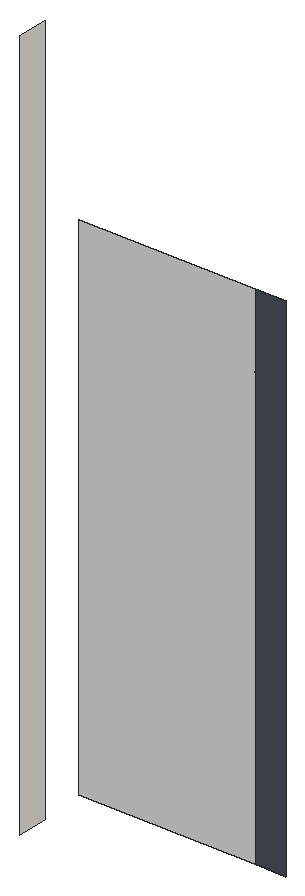
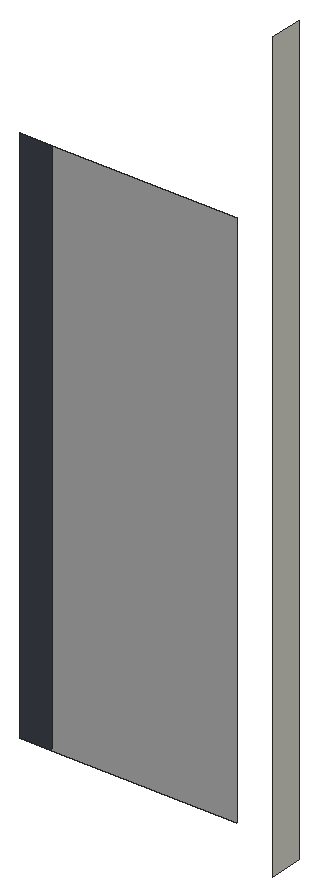
# SketchUp Ruby script. Lengths in inches.
U = 1.inch
M = Sketchup.active_model
def pt(a) = Geom::Point3d.new(a.map { |v| v * U })
def face(e, loops, mat)
  f = e.add_face(loops[0].map { |a| pt(a) })
  loops[1..].each { |l| e.add_face(l.map { |a| pt(a) }).erase! }
  f.material = f.back_material = mat if mat
  f
end
# faces: each face lists its corners as indices into pts; further lists are holes
def faces(e, pts, list, mat = nil) = list.each { |f| face(e, (f[0].is_a?(Array) ? f : [f]).map { |l| l.map { |i| pts[i] } }, mat) }
# xy, xz, yz: faces in a plane at the given z, y or x. An outline is a flat list of corners, or four numbers for a rectangle; further outlines are holes
def ring(l) = l.size == 4 ? [[l[0], l[1]], [l[2], l[1]], [l[2], l[3]], [l[0], l[3]]] : l.each_slice(2).to_a
def flat(e, list, mat, &to3) = list.each { |f| face(e, (f[0].is_a?(Array) ? f : [f]).map { |l| ring(l).map { |u, v| to3.(u, v) } }, mat) }
def xy(e, z, list, mat = nil) = flat(e, list, mat) { |x, y| [x, y, z] }
def xz(e, y, list, mat = nil) = flat(e, list, mat) { |x, z| [x, y, z] }
def yz(e, x, list, mat = nil) = flat(e, list, mat) { |y, z| [x, y, z] }
def lines(e, pts, list) = list.each { |a, b| e.add_line(pt(pts[a]), pt(pts[b])) }
# prism: a flat outline (further loops are holes) pulled along v
def prism(e, loops, v, mat = nil)
  f = face(e, loops, mat); d = Geom::Vector3d.new(v.map { |x| x * U })
  f.pushpull(f.normal.samedirection?(d) ? d.length : -d.length)
end
def box(e, o, s, mat = nil) = prism(e, [[o, [o[0] + s[0], o[1], o[2]], [o[0] + s[0], o[1] + s[1], o[2]], [o[0], o[1] + s[1], o[2]]]], [0, 0, s[2]], mat)
def at(x, y, z, deg = 0) = Geom::Transformation.translation(pt([x, y, z])) * Geom::Transformation.rotation(ORIGIN, Z_AXIS, deg.degrees)
def axes(o, x, y, z) = Geom::Transformation.new([*x, 0, *y, 0, *z, 0, *pt(o).to_a, 1])
def part(name) = M.definitions.add(name)
# library, detail: a bought-in or finely detailed component or shape, given as its bounding box
def library(name, o, s) = part(name).tap { |d| box(d.entities, o, s) }
def detail(e, o, s) = box(e.add_group.entities, o, s)
def put(e, d, t, mat = nil) = e.add_instance(d, t).tap { |i| i.material = mat if mat }
def group(e, t, mat = nil) = e.add_group.tap { |g| g.transformation = t; g.material = mat if mat }.entities
root = M.entities
M.materials.add("[Formica Laminate Dark]").color = [74, 78, 89]
M.materials.add("[Mirror 01]").color = [216, 216, 216]
M.materials.add("[Tile Limestone Large]").color = [237, 234, 224]
xz(root,244.48,[[183.37,96.33,193.875,272.12]],"[Formica Laminate Dark]")
xz(root,244.48,[[123.4,96.33,183.37,272.12]],"[Mirror 01]")
yz(root,111.93,[[233.86,84.87,244.48,328.93]],"[Tile Limestone Large]")
